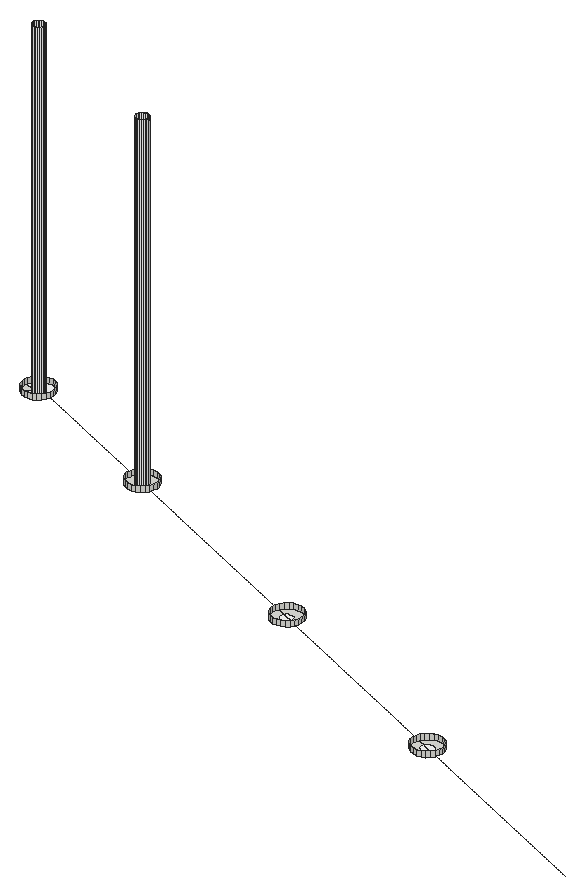
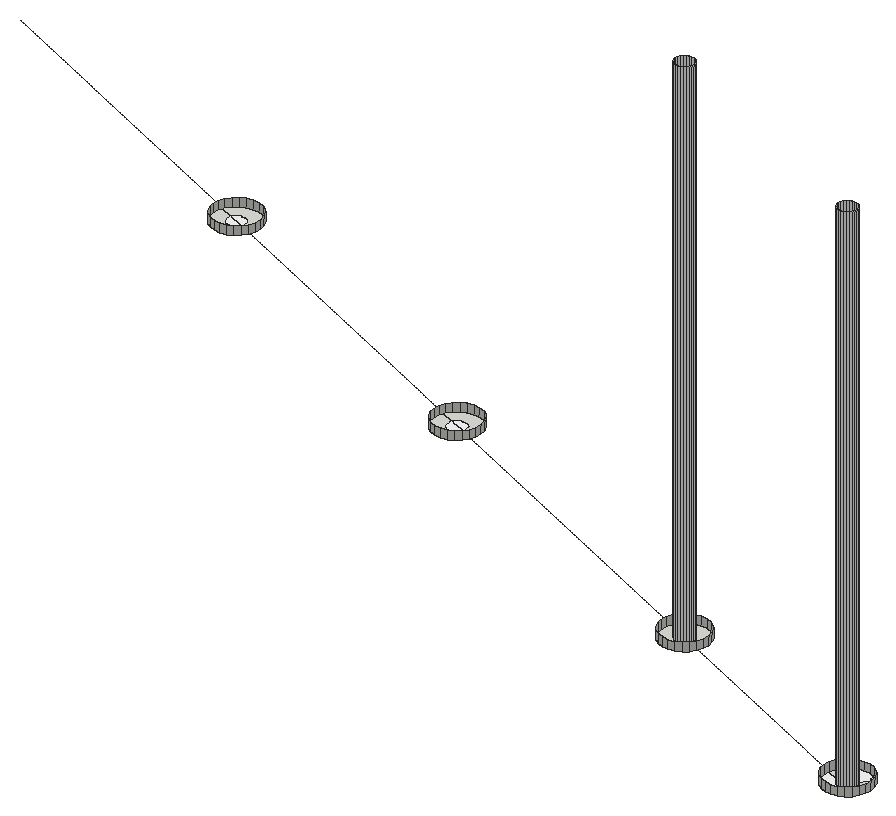
# SketchUp Ruby script. Lengths in inches.
U = 1.inch
M = Sketchup.active_model
def pt(a) = Geom::Point3d.new(a.map { |v| v * U })
def face(e, loops, mat)
  f = e.add_face(loops[0].map { |a| pt(a) })
  loops[1..].each { |l| e.add_face(l.map { |a| pt(a) }).erase! }
  f.material = f.back_material = mat if mat
  f
end
# faces: each face lists its corners as indices into pts; further lists are holes
def faces(e, pts, list, mat = nil) = list.each { |f| face(e, (f[0].is_a?(Array) ? f : [f]).map { |l| l.map { |i| pts[i] } }, mat) }
# xy, xz, yz: faces in a plane at the given z, y or x. An outline is a flat list of corners, or four numbers for a rectangle; further outlines are holes
def ring(l) = l.size == 4 ? [[l[0], l[1]], [l[2], l[1]], [l[2], l[3]], [l[0], l[3]]] : l.each_slice(2).to_a
def flat(e, list, mat, &to3) = list.each { |f| face(e, (f[0].is_a?(Array) ? f : [f]).map { |l| ring(l).map { |u, v| to3.(u, v) } }, mat) }
def xy(e, z, list, mat = nil) = flat(e, list, mat) { |x, y| [x, y, z] }
def xz(e, y, list, mat = nil) = flat(e, list, mat) { |x, z| [x, y, z] }
def yz(e, x, list, mat = nil) = flat(e, list, mat) { |y, z| [x, y, z] }
def lines(e, pts, list) = list.each { |a, b| e.add_line(pt(pts[a]), pt(pts[b])) }
# prism: a flat outline (further loops are holes) pulled along v
def prism(e, loops, v, mat = nil)
  f = face(e, loops, mat); d = Geom::Vector3d.new(v.map { |x| x * U })
  f.pushpull(f.normal.samedirection?(d) ? d.length : -d.length)
end
def box(e, o, s, mat = nil) = prism(e, [[o, [o[0] + s[0], o[1], o[2]], [o[0] + s[0], o[1] + s[1], o[2]], [o[0], o[1] + s[1], o[2]]]], [0, 0, s[2]], mat)
def at(x, y, z, deg = 0) = Geom::Transformation.translation(pt([x, y, z])) * Geom::Transformation.rotation(ORIGIN, Z_AXIS, deg.degrees)
def axes(o, x, y, z) = Geom::Transformation.new([*x, 0, *y, 0, *z, 0, *pt(o).to_a, 1])
def part(name) = M.definitions.add(name)
# library, detail: a bought-in or finely detailed component or shape, given as its bounding box
def library(name, o, s) = part(name).tap { |d| box(d.entities, o, s) }
def detail(e, o, s) = box(e.add_group.entities, o, s)
def put(e, d, t, mat = nil) = e.add_instance(d, t).tap { |i| i.material = mat if mat }
def group(e, t, mat = nil) = e.add_group.tap { |g| g.transformation = t; g.material = mat if mat }.entities
root = M.entities
M.materials.add("[Color_000]").color = [255, 255, 255]
xy(root,321.267,[[824.098,1097.975,823.6875,1098,823.298,1098.13,822.954,1098.356,822.681,1098.663,822.497,1099.031,822.415,1099.434,822.439,1099.844,822.548,1100.172,823.411,1099.797,823.367,1099.665,823.357,1099.501,823.39,1099.34,823.464,1099.193,823.573,1099.07,823.71,1098.98,823.866,1098.928,824.03,1098.918,824.192,1098.951,824.339,1099.025,824.462,1099.134,824.552,1099.271,824.56,1099.296,825.423,1098.92,825.402,1098.858,825.176,1098.515,824.868,1098.242,824.501,1098.058],[[824.098,1097.975,824.501,1098.058,824.868,1098.242,825.176,1098.515,825.402,1098.858,825.423,1098.92,825.532,1099.248,825.556,1099.659,825.474,1100.062,825.289,1100.429,825.017,1100.737,824.673,1100.963,824.283,1101.093,823.873,1101.117,823.47,1101.034,823.103,1100.85,822.795,1100.577,822.569,1100.234,822.548,1100.172,822.439,1099.844,822.415,1099.434,822.497,1099.031,822.681,1098.663,822.954,1098.356,823.298,1098.13,823.6875,1098],[824.03,1098.918,823.866,1098.928,823.71,1098.98,823.573,1099.07,823.464,1099.193,823.39,1099.34,823.357,1099.501,823.367,1099.665,823.419,1099.821,823.509,1099.959,823.632,1100.068,823.779,1100.142,823.94,1100.175,824.105,1100.165,824.261,1100.113,824.398,1100.022,824.507,1099.899,824.581,1099.752,824.614,1099.591,824.604,1099.427,824.56,1099.296,824.552,1099.271,824.462,1099.134,824.339,1099.025,824.192,1098.951]],[800.488,1108.258,800.078,1108.283,799.6875,1108.412,799.344,1108.639,799.072,1108.946,798.887,1109.314,798.805,1109.716,798.829,1110.127,798.938,1110.455,799.801,1110.079,799.757,1109.948,799.747,1109.784,799.78,1109.623,799.854,1109.476,799.963,1109.353,800.1,1109.262,800.256,1109.211,800.421,1109.201,800.582,1109.234,800.729,1109.307,800.852,1109.417,800.942,1109.554,800.95,1109.579,801.813,1109.203,801.792,1109.141,801.566,1108.798,801.258,1108.525,800.891,1108.341],[[800.488,1108.258,800.078,1108.283,799.6875,1108.412,799.344,1108.639,799.072,1108.946,798.887,1109.314,798.805,1109.716,798.829,1110.127,798.938,1110.455,798.959,1110.517,799.185,1110.86,799.493,1111.133,799.86,1111.317,800.263,1111.4,800.673,1111.375,801.063,1111.246,801.407,1111.019,801.68,1110.712,801.864,1110.344,801.946,1109.942,801.922,1109.531,801.813,1109.203,801.792,1109.141,801.566,1108.798,801.258,1108.525,800.891,1108.341],[800.421,1109.201,800.582,1109.234,800.729,1109.307,800.852,1109.417,800.942,1109.554,800.95,1109.579,800.994,1109.71,801.004,1109.874,800.971,1110.035,800.897,1110.182,800.788,1110.305,800.651,1110.396,800.495,1110.448,800.331,1110.457,800.169,1110.424,800.022,1110.351,799.899,1110.242,799.809,1110.104,799.801,1110.079,799.757,1109.948,799.747,1109.784,799.78,1109.623,799.854,1109.476,799.963,1109.353,800.1,1109.262,800.256,1109.211]],[[776.144,1118.861,775.734,1118.885,775.344,1119.015,775,1119.241,774.728,1119.549,774.543,1119.916,774.461,1120.319,774.485,1120.729,774.594,1121.058,774.615,1121.12,774.841,1121.463,775.149,1121.736,775.516,1121.92,775.919,1122.002,776.329,1121.978,776.719,1121.848,777.0625,1121.622,777.336,1121.315,777.52,1120.947,777.602,1120.544,777.578,1120.134,777.469,1119.806,777.448,1119.744,777.222,1119.401,776.914,1119.128,776.547,1118.944],[776.077,1119.803,776.238,1119.836,776.385,1119.91,776.508,1120.019,776.598,1120.156,776.606,1120.181,776.65,1120.3125,776.66,1120.477,776.627,1120.638,776.553,1120.785,776.444,1120.908,776.307,1120.998,776.151,1121.05,775.987,1121.06,775.825,1121.027,775.678,1120.953,775.555,1120.844,775.465,1120.707,775.457,1120.682,775.413,1120.551,775.403,1120.387,775.436,1120.226,775.51,1120.078,775.619,1119.956,775.756,1119.865,775.912,1119.813]],
  [776.077,1119.803,776.238,1119.836,776.385,1119.91,776.508,1120.019,776.598,1120.156,776.606,1120.181,775.457,1120.682,775.413,1120.551,775.403,1120.387,775.436,1120.226,775.51,1120.078,775.619,1119.956,775.756,1119.865,775.912,1119.813],[759.3125,1125.943,759.556,1125.993,759.924,1126.177,760.231,1126.45,760.458,1126.793,760.58,1127.161,760.351,1127.261,759.983,1127.407,759.895,1127.436,759.806,1127.458,759.716,1127.475,759.667,1127.48,759.66,1127.362,759.608,1127.206,759.517,1127.069,759.394,1126.96,759.247,1126.886,759.09,1126.854,759.242,1126.551,759.325,1126.148],[758.381,1126.056,758.353,1126.065,758.046,1126.267,758.092,1126.373,758.16,1126.516,758.166,1126.512,758.276,1126.389,758.349,1126.242,758.382,1126.081],[758.16,1126.516,758.262,1126.731,758.306,1126.811,758.356,1126.888,758.411,1126.961,758.47,1127.031,758.534,1127.097,758.541,1127.103,758.519,1127.128,758.446,1127.275,758.413,1127.436,758.414,1127.462,758.052,1127.582,757.641,1127.607,757.483,1127.574,757.47,1127.369,757.553,1126.966,757.705,1126.663,757.709,1126.664,757.873,1126.654,758.029,1126.602],[759.086,1126.853,759.09,1126.854,759.058,1126.919,758.785,1127.226,758.736,1127.258,758.674,1127.216,758.602,1127.159,758.541,1127.103,758.629,1127.005,758.766,1126.915,758.922,1126.863]])
xy(root,321.267,[[824.03,1098.918,823.866,1098.928,823.71,1098.98,823.573,1099.07,823.464,1099.193,823.39,1099.34,823.357,1099.501,823.367,1099.665,823.411,1099.797,824.56,1099.296,824.552,1099.271,824.462,1099.134,824.339,1099.025,824.192,1098.951],[824.56,1099.296,823.411,1099.797,823.419,1099.821,823.509,1099.959,823.632,1100.068,823.779,1100.142,823.94,1100.175,824.105,1100.165,824.261,1100.113,824.398,1100.022,824.507,1099.899,824.581,1099.752,824.614,1099.591,824.604,1099.427],[800.421,1109.201,800.256,1109.211,800.1,1109.262,799.963,1109.353,799.854,1109.476,799.78,1109.623,799.747,1109.784,799.757,1109.948,799.801,1110.079,800.95,1109.579,800.942,1109.554,800.852,1109.417,800.729,1109.307,800.582,1109.234],[800.95,1109.579,799.801,1110.079,799.809,1110.104,799.899,1110.242,800.022,1110.351,800.169,1110.424,800.331,1110.457,800.495,1110.448,800.651,1110.396,800.788,1110.305,800.897,1110.182,800.971,1110.035,801.004,1109.874,800.994,1109.71],[776.144,1118.861,775.734,1118.885,775.344,1119.015,775,1119.241,774.728,1119.549,774.543,1119.916,774.461,1120.319,774.485,1120.729,774.594,1121.058,775.457,1120.682,775.413,1120.551,775.403,1120.387,775.436,1120.226,775.51,1120.078,775.619,1119.956,775.756,1119.865,775.912,1119.813,776.077,1119.803,776.238,1119.836,776.385,1119.91,776.508,1120.019,776.598,1120.156,776.606,1120.181,777.469,1119.806,777.448,1119.744,777.222,1119.401,776.914,1119.128,776.547,1118.944],
  [776.606,1120.181,775.457,1120.682,775.465,1120.707,775.555,1120.844,775.678,1120.953,775.825,1121.027,775.987,1121.06,776.151,1121.05,776.307,1120.998,776.444,1120.908,776.553,1120.785,776.627,1120.638,776.66,1120.477,776.65,1120.3125],[759.154,1125.911,758.743,1125.935,758.381,1126.056,758.382,1126.081,758.349,1126.242,758.276,1126.389,758.166,1126.512,758.16,1126.516,758.262,1126.731,758.306,1126.811,758.356,1126.888,758.411,1126.961,758.47,1127.031,758.534,1127.097,758.541,1127.103,758.629,1127.005,758.766,1126.915,758.922,1126.863,759.086,1126.853,759.09,1126.854,759.242,1126.551,759.325,1126.148,759.3125,1125.943],[758.046,1126.267,758.01,1126.291,757.737,1126.598,757.705,1126.663,757.709,1126.664,757.873,1126.654,758.029,1126.602,758.16,1126.516,758.092,1126.373],[759.09,1126.854,759.058,1126.919,758.785,1127.226,758.736,1127.258,758.75,1127.268,758.829,1127.315,758.911,1127.356,758.995,1127.393,759.081,1127.424,759.17,1127.449,759.259,1127.468,759.35,1127.481,759.442,1127.488,759.533,1127.49,759.625,1127.485,759.667,1127.48,759.66,1127.362,759.608,1127.206,759.517,1127.069,759.394,1126.96,759.247,1126.886],[758.541,1127.103,758.519,1127.128,758.446,1127.275,758.413,1127.436,758.414,1127.462,758.442,1127.452,758.736,1127.258,758.674,1127.216,758.602,1127.159],
  [760.58,1127.161,760.351,1127.261,759.983,1127.407,759.895,1127.436,759.806,1127.458,759.716,1127.475,759.667,1127.48,759.669,1127.526,759.636,1127.6875,759.563,1127.834,759.454,1127.957,759.316,1128.048,759.16,1128.1,758.996,1128.11,758.835,1128.077,758.688,1128.003,758.565,1127.894,758.474,1127.756,758.423,1127.6,758.414,1127.462,758.052,1127.582,757.641,1127.607,757.483,1127.574,757.495,1127.779,757.624,1128.169,757.851,1128.512,758.158,1128.785,758.526,1128.969,758.929,1129.052,759.339,1129.028,759.729,1128.898,760.072,1128.672,760.345,1128.364,760.529,1127.997,760.612,1127.594,760.587,1127.184],[758.736,1127.258,758.75,1127.268,758.829,1127.315,758.911,1127.356,758.995,1127.393,759.081,1127.424,759.17,1127.449,759.259,1127.468,759.35,1127.481,759.442,1127.488,759.533,1127.49,759.625,1127.485,759.667,1127.48,759.669,1127.526,759.636,1127.6875,759.563,1127.834,759.454,1127.957,759.316,1128.048,759.16,1128.1,758.996,1128.11,758.835,1128.077,758.688,1128.003,758.565,1127.894,758.474,1127.756,758.423,1127.6,758.414,1127.462,758.442,1127.452]],"[Color_000]")
p = [[823.298,1098.13,321.267],[823.6875,1098,321.267],[823.6875,1098,321.858],[823.298,1098.13,321.858],[824.098,1097.975,321.267],[824.098,1097.975,321.858],
  [824.501,1098.058,321.267],[824.501,1098.058,321.858],[822.954,1098.356,321.267],[822.954,1098.356,321.858],[824.868,1098.242,321.267],[824.868,1098.242,321.858],
  [825.176,1098.515,321.267],[825.176,1098.515,321.858],[822.681,1098.663,321.267],[822.681,1098.663,321.858],[825.402,1098.858,321.267],[825.402,1098.858,321.858],
  [822.497,1099.031,321.267],[822.497,1099.031,321.858],[825.423,1098.92,321.267],[825.532,1099.248,321.267],[825.532,1099.248,321.858],[822.415,1099.434,321.267],
  [822.415,1099.434,321.858],[825.556,1099.659,321.267],[825.556,1099.659,321.858],[822.439,1099.844,321.267],[822.439,1099.844,321.858],[825.474,1100.062,321.267],
  [825.474,1100.062,321.858],[822.569,1100.234,321.267],[822.548,1100.172,321.267],[822.569,1100.234,321.858],[825.289,1100.429,321.267],[825.289,1100.429,321.858],
  [822.795,1100.577,321.267],[822.795,1100.577,321.858],[825.017,1100.737,321.267],[825.017,1100.737,321.858],[823.103,1100.85,321.267],[823.103,1100.85,321.858],
  [824.673,1100.963,321.267],[824.673,1100.963,321.858],[823.47,1101.034,321.267],[823.47,1101.034,321.858],[823.873,1101.117,321.267],[823.873,1101.117,321.858],
  [824.283,1101.093,321.267],[824.283,1101.093,321.858],[799.6875,1108.412,321.267],[800.078,1108.283,321.267],[800.078,1108.283,321.858],[799.6875,1108.412,321.858],
  [800.488,1108.258,321.267],[800.488,1108.258,321.858],[800.891,1108.341,321.267],[800.891,1108.341,321.858],[801.258,1108.525,321.267],[801.258,1108.525,321.858],
  [799.344,1108.639,321.267],[799.344,1108.639,321.858],[801.566,1108.798,321.267],[801.566,1108.798,321.858],[799.072,1108.946,321.267],[799.072,1108.946,321.858],
  [801.792,1109.141,321.267],[801.792,1109.141,321.858],[798.887,1109.314,321.267],[798.887,1109.314,321.858],[801.813,1109.203,321.267],[801.922,1109.531,321.267],
  [801.922,1109.531,321.858],[798.805,1109.716,321.267],[798.805,1109.716,321.858],[801.946,1109.942,321.267],[801.946,1109.942,321.858],[798.829,1110.127,321.267],
  [798.829,1110.127,321.858],[801.864,1110.344,321.267],[801.864,1110.344,321.858],[798.959,1110.517,321.267],[798.938,1110.455,321.267],[798.959,1110.517,321.858],
  [801.68,1110.712,321.267],[801.68,1110.712,321.858],[799.185,1110.86,321.267],[799.185,1110.86,321.858],[801.407,1111.019,321.267],[801.407,1111.019,321.858],
  [799.493,1111.133,321.267],[799.493,1111.133,321.858],[801.063,1111.246,321.267],[801.063,1111.246,321.858],[799.86,1111.317,321.267],[799.86,1111.317,321.858],
  [800.673,1111.375,321.267],[800.673,1111.375,321.858],[800.263,1111.4,321.267],[800.263,1111.4,321.858],[775.344,1119.015,321.267],[775.734,1118.885,321.267],
  [775.734,1118.885,321.858],[775.344,1119.015,321.858],[776.144,1118.861,321.267],[776.144,1118.861,321.858],[776.547,1118.944,321.267],[776.547,1118.944,321.858],
  [776.914,1119.128,321.267],[776.914,1119.128,321.858],[775,1119.241,321.267],[775,1119.241,321.858],[777.222,1119.401,321.267],[777.222,1119.401,321.858],
  [774.728,1119.549,321.267],[774.728,1119.549,321.858],[777.448,1119.744,321.267],[777.448,1119.744,321.858],[774.543,1119.916,321.267],[774.543,1119.916,321.858],
  [777.469,1119.806,321.267],[777.578,1120.134,321.267],[777.578,1120.134,321.858],[775.756,1119.865,321.267],[775.912,1119.813,321.267],[775.912,1119.813,357.267],
  [775.756,1119.865,357.267],[776.077,1119.803,321.267],[776.077,1119.803,357.267],[776.238,1119.836,321.267],[776.238,1119.836,357.267],[776.385,1119.91,321.267],
  [776.385,1119.91,357.267],[774.461,1120.319,321.267],[774.461,1120.319,321.858],[775.619,1119.956,321.267],[775.619,1119.956,357.267],[776.508,1120.019,321.267],
  [776.508,1120.019,357.267],[775.51,1120.078,321.267],[775.51,1120.078,357.267],[776.598,1120.156,321.267],[776.598,1120.156,357.267],[775.436,1120.226,321.267],
  [775.436,1120.226,357.267],[777.602,1120.544,321.267],[777.602,1120.544,321.858],[775.403,1120.387,321.267],[775.403,1120.387,357.267],[776.606,1120.181,321.267],
  [776.65,1120.3125,321.267],[776.65,1120.3125,357.267],[774.485,1120.729,321.267],[774.485,1120.729,321.858],[776.66,1120.477,321.267],[776.66,1120.477,357.267],
  [775.413,1120.551,321.267],[775.413,1120.551,357.267],[776.627,1120.638,321.267],[776.627,1120.638,357.267],[777.52,1120.947,321.267],[777.52,1120.947,321.858],
  [775.465,1120.707,321.267],[775.457,1120.682,321.267],[775.465,1120.707,357.267],[776.553,1120.785,321.267],[776.553,1120.785,357.267],[774.615,1121.12,321.267],
  [774.594,1121.058,321.267],[774.615,1121.12,321.858],[775.555,1120.844,321.267],[775.555,1120.844,357.267],[775.678,1120.953,321.267],[775.678,1120.953,357.267],
  [776.444,1120.908,321.267],[776.444,1120.908,357.267],[776.307,1120.998,321.267],[776.307,1120.998,357.267],[777.336,1121.315,321.267],[777.336,1121.315,321.858],
  [775.825,1121.027,321.267],[775.825,1121.027,357.267],[775.987,1121.06,321.267],[775.987,1121.06,357.267],[776.151,1121.05,321.267],[776.151,1121.05,357.267],
  [774.841,1121.463,321.267],[774.841,1121.463,321.858],[777.0625,1121.622,321.267],[777.0625,1121.622,321.858],[775.149,1121.736,321.267],[775.149,1121.736,321.858],
  [776.719,1121.848,321.267],[776.719,1121.848,321.858],[775.516,1121.92,321.267],[775.516,1121.92,321.858],[776.329,1121.978,321.267],[776.329,1121.978,321.858],
  [775.919,1122.002,321.267],[775.919,1122.002,321.858],[758.353,1126.065,321.267],[758.381,1126.056,321.267],[758.743,1125.935,321.267],[758.743,1125.935,321.858],
  [758.353,1126.065,321.858],[759.154,1125.911,321.267],[759.154,1125.911,321.858],[759.3125,1125.943,321.267],[759.556,1125.993,321.267],[759.556,1125.993,321.858],
  [759.3125,1125.943,321.858],[759.924,1126.177,321.267],[759.924,1126.177,321.858],[758.01,1126.291,321.267],[758.046,1126.267,321.267],[758.01,1126.291,321.858],
  [760.231,1126.45,321.267],[760.231,1126.45,321.858],[757.737,1126.598,321.267],[757.737,1126.598,321.858],[760.458,1126.793,321.267],[760.458,1126.793,321.858],
  [757.553,1126.966,321.267],[757.705,1126.663,321.267],[757.553,1126.966,321.858],[760.58,1127.161,321.267],[760.587,1127.184,321.267],[760.587,1127.184,321.858],
  [758.629,1127.005,321.267],[758.766,1126.915,321.267],[758.766,1126.915,357.267],[758.629,1127.005,357.267],[758.922,1126.863,321.267],[758.922,1126.863,357.267],
  [759.086,1126.853,321.267],[759.086,1126.853,357.267],[759.09,1126.854,321.267],[759.247,1126.886,321.267],[759.247,1126.886,357.267],[759.394,1126.96,321.267],
  [759.394,1126.96,357.267],[757.47,1127.369,321.267],[757.47,1127.369,321.858],[758.519,1127.128,321.267],[758.541,1127.103,321.267],[758.519,1127.128,357.267],
  [759.517,1127.069,321.267],[759.517,1127.069,357.267],[758.446,1127.275,321.267],[758.446,1127.275,357.267],[759.608,1127.206,321.267],[759.608,1127.206,357.267],
  [759.66,1127.362,321.267],[759.66,1127.362,357.267],[760.612,1127.594,321.267],[760.612,1127.594,321.858],[758.413,1127.436,321.267],[758.413,1127.436,357.267],
  [757.495,1127.779,321.267],[757.483,1127.574,321.267],[757.483,1127.574,321.858],[757.495,1127.779,321.858],[758.423,1127.6,321.267],[758.414,1127.462,321.267],
  [758.423,1127.6,357.267],[759.667,1127.48,321.267],[759.669,1127.526,321.267],[759.669,1127.526,357.267],[759.636,1127.6875,321.267],[759.636,1127.6875,357.267],
  [758.474,1127.756,321.267],[758.474,1127.756,357.267],[760.529,1127.997,321.267],[760.529,1127.997,321.858],[759.563,1127.834,321.267],[759.563,1127.834,357.267],
  [757.624,1128.169,321.267],[757.624,1128.169,321.858],[758.565,1127.894,321.267],[758.565,1127.894,357.267],[759.454,1127.957,321.267],[759.454,1127.957,357.267],
  [758.688,1128.003,321.267],[758.688,1128.003,357.267],[758.835,1128.077,321.267],[758.835,1128.077,357.267],[759.316,1128.048,321.267],[759.16,1128.1,321.267],
  [759.16,1128.1,357.267],[759.316,1128.048,357.267],[760.345,1128.364,321.267],[760.345,1128.364,321.858],[758.996,1128.11,321.267],[758.996,1128.11,357.267],
  [757.851,1128.512,321.267],[757.851,1128.512,321.858],[760.072,1128.672,321.267],[760.072,1128.672,321.858],[758.158,1128.785,321.267],[758.158,1128.785,321.858],
  [759.729,1128.898,321.267],[759.729,1128.898,321.858],[758.526,1128.969,321.267],[758.526,1128.969,321.858],[759.339,1129.028,321.267],[759.339,1129.028,321.858],
  [758.929,1129.052,321.267],[758.929,1129.052,321.858],[847.132,1089.465,321.267]]
faces(root,p,[[0,1,2,3],[1,4,5,2],[4,6,7,5],[8,0,3,9],[6,10,11,7],[10,12,13,11],[14,8,9,15],[12,16,17,13],
  [18,14,15,19],[16,20,21,22,17],[23,18,19,24],[21,25,26,22],[27,23,24,28],[25,29,30,26],[31,32,27,28,33],[29,34,35,30],
  [36,31,33,37],[34,38,39,35],[40,36,37,41],[38,42,43,39],[44,40,41,45],[46,44,45,47],[42,48,49,43],[48,46,47,49],
  [50,51,52,53],[51,54,55,52],[54,56,57,55],[56,58,59,57],[60,50,53,61],[58,62,63,59],[64,60,61,65],[62,66,67,63],
  [68,64,65,69],[66,70,71,72,67],[73,68,69,74],[71,75,76,72],[77,73,74,78],[75,79,80,76],[81,82,77,78,83],[79,84,85,80],
  [86,81,83,87],[84,88,89,85],[90,86,87,91],[88,92,93,89],[94,90,91,95],[92,96,97,93],[98,94,95,99],[96,98,99,97],
  [100,101,102,103],[101,104,105,102],[104,106,107,105],[106,108,109,107],[110,100,103,111],[108,112,113,109],[114,110,111,115],[112,116,117,113],
  [118,114,115,119],[116,120,121,122,117],[133,118,119,134],[121,145,146,122],[152,133,134,153],[145,160,161,146],[167,168,152,153,169],[160,178,179,161],
  [186,167,169,187],[178,188,189,179],[190,186,187,191],[188,192,193,189],[194,190,191,195],[192,196,197,193],[198,194,195,199],[196,198,199,197],
  [200,201,202,203,204],[202,205,206,203],[205,207,208,209,210,206],[208,211,212,209],[213,214,200,204,215],[211,216,217,212],[218,213,215,219],[216,220,221,217],
  [222,223,218,219,224],[220,225,226,227,221],[241,222,224,242],[226,254,255,227],[258,259,241,242,260,261],[254,272,273,255],[276,258,261,277],[272,290,291,273],
  [294,276,277,295],[290,296,297,291],[298,294,295,299],[296,300,301,297],[302,298,299,303],[300,304,305,301],[306,302,303,307],[304,306,307,305]])
faces(root,p,[[123,124,125,126],[124,127,128,125],[127,129,130,128],[129,131,132,130],[135,123,126,136],[131,137,138,132],[139,135,136,140],[137,141,142,138],
  [143,139,140,144],[147,143,144,148],[141,149,150,151,142],[150,154,155,151],[156,147,148,157],[154,158,159,155],[162,163,156,157,164],[158,165,166,159],
  [170,162,164,171],[172,170,171,173],[165,174,175,166],[174,176,177,175],[180,172,173,181],[182,180,181,183],[176,184,185,177],[184,182,183,185],
  [228,229,230,231],[229,232,233,230],[232,234,235,233],[234,236,237,238,235],[237,239,240,238],[243,244,228,231,245],[239,246,247,240],[248,243,245,249],
  [246,250,251,247],[250,252,253,251],[256,248,249,257],[262,263,256,257,264],[252,265,266,267,253],[266,268,269,267],[270,262,264,271],[268,274,275,269],
  [278,270,271,279],[274,280,281,275],[282,278,279,283],[284,282,283,285],[286,287,288,289],[280,286,289,281],[292,284,285,293],[287,292,293,288]],"[Color_000]")
lines(root,p,[[308,20],[32,70],[82,120],[168,225]])
